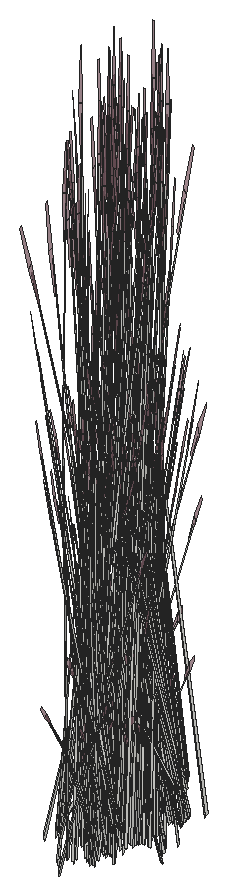
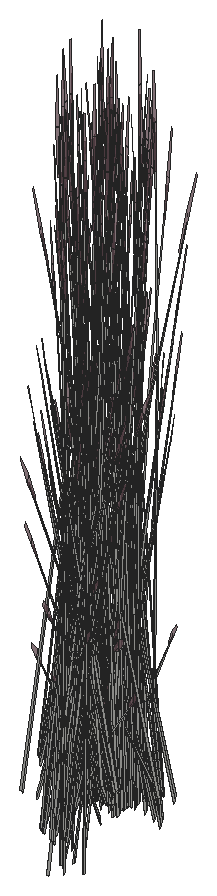
# SketchUp Ruby script. Lengths in inches.
U = 1.inch
M = Sketchup.active_model
def pt(a) = Geom::Point3d.new(a.map { |v| v * U })
def face(e, loops, mat)
  f = e.add_face(loops[0].map { |a| pt(a) })
  loops[1..].each { |l| e.add_face(l.map { |a| pt(a) }).erase! }
  f.material = f.back_material = mat if mat
  f
end
# faces: each face lists its corners as indices into pts; further lists are holes
def faces(e, pts, list, mat = nil) = list.each { |f| face(e, (f[0].is_a?(Array) ? f : [f]).map { |l| l.map { |i| pts[i] } }, mat) }
# xy, xz, yz: faces in a plane at the given z, y or x. An outline is a flat list of corners, or four numbers for a rectangle; further outlines are holes
def ring(l) = l.size == 4 ? [[l[0], l[1]], [l[2], l[1]], [l[2], l[3]], [l[0], l[3]]] : l.each_slice(2).to_a
def flat(e, list, mat, &to3) = list.each { |f| face(e, (f[0].is_a?(Array) ? f : [f]).map { |l| ring(l).map { |u, v| to3.(u, v) } }, mat) }
def xy(e, z, list, mat = nil) = flat(e, list, mat) { |x, y| [x, y, z] }
def xz(e, y, list, mat = nil) = flat(e, list, mat) { |x, z| [x, y, z] }
def yz(e, x, list, mat = nil) = flat(e, list, mat) { |y, z| [x, y, z] }
def lines(e, pts, list) = list.each { |a, b| e.add_line(pt(pts[a]), pt(pts[b])) }
# prism: a flat outline (further loops are holes) pulled along v
def prism(e, loops, v, mat = nil)
  f = face(e, loops, mat); d = Geom::Vector3d.new(v.map { |x| x * U })
  f.pushpull(f.normal.samedirection?(d) ? d.length : -d.length)
end
def box(e, o, s, mat = nil) = prism(e, [[o, [o[0] + s[0], o[1], o[2]], [o[0] + s[0], o[1] + s[1], o[2]], [o[0], o[1] + s[1], o[2]]]], [0, 0, s[2]], mat)
def at(x, y, z, deg = 0) = Geom::Transformation.translation(pt([x, y, z])) * Geom::Transformation.rotation(ORIGIN, Z_AXIS, deg.degrees)
def axes(o, x, y, z) = Geom::Transformation.new([*x, 0, *y, 0, *z, 0, *pt(o).to_a, 1])
def part(name) = M.definitions.add(name)
# library, detail: a bought-in or finely detailed component or shape, given as its bounding box
def library(name, o, s) = part(name).tap { |d| box(d.entities, o, s) }
def detail(e, o, s) = box(e.add_group.entities, o, s)
def put(e, d, t, mat = nil) = e.add_instance(d, t).tap { |i| i.material = mat if mat }
def group(e, t, mat = nil) = e.add_group.tap { |g| g.transformation = t; g.material = mat if mat }.entities
root = M.entities
M.materials.add("LightPink_Translucent").color = [144, 107, 117]
M.materials["LightPink_Translucent"].alpha = 0.75
c1 = part("blade")
p = [[2.15,0.21,22],[0,0.17,0],[0.09,0.45,0],[2.18,0.31,22],[2.29,0.31,22],[0.38,0.45,0],
  [2.48,0.24,33],[2.49,0.24,33],[2.48,0.22,33]]
faces(c1.entities,p,[[0,1,2,3],[4,5,2,3],[6,3,4,7],[8,0,3,6]])
c2 = part("seeds")
p = [[0.3,-0.1,1.38],[-0.01,-0.03,1.59],[-0.01,-0.03,0.03],[0.14,-0.07,-0.07],[0.29,-0.03,3],[0.15,0.01,3.11]]
faces(c2.entities,p,[[0,1,2,3],[1,0,4,5]],"LightPink_Translucent")
c3 = part("blade with seeds")
put(c3.entities,c1,at(0,0,0))
put(c3.entities,c2,axes([2.4,0.25,30.99],[1.5799,-0.05474,1.17369],[-0.12525,1.92788,0.29478],[-0.07173,-0.02425,1.56792]))
put(root,c3,axes([358.98,656.59,622.9],[-0.23773,0.35053,-0.62353],[-0.29532,-0.31785,-0.16365],[-0.09526,0.08744,1.37633]))
put(root,c3,axes([357.93,660.52,622.73],[0.16041,-0.29625,0.0643],[0.22843,0.17248,0.50621],[-0.07385,-0.09498,0.77189]))
put(root,c3,axes([358.37,653.98,625.9],[0.05451,0.37564,0.35414],[-0.31161,0.09919,-0.4572],[-0.0837,-0.10765,0.87481]))
put(root,c3,axes([357.79,654.2,622.64],[-0.2773,-0.3397,0.17642],[0.27945,-0.32949,0.35086],[-0.03063,0.06937,1.60407]))
put(root,c3,axes([357.66,655.44,623.18],[-0.32829,0.39208,0.30756],[-0.32849,-0.38796,-0.36492],[-0.01146,-0.11134,1.64885]))
put(root,c3,axes([356.83,654,622.375],[0,-0.53961,0],[0.44133,0,0],[0,0,1.79456]))
put(root,c3,axes([356.42,654.1,622.6],[0.39767,0.22603,0.24065],[-0.19139,0.46966,0.50002],[0,-0.10827,1.60543]))
put(root,c3,axes([357.05,654.22,622.46],[0,0.53934,-0.05637],[-0.44133,0,0],[0,0.01695,1.79368]))
put(root,c3,axes([359.01,656.53,624.17],[0.305,0.18805,1.51261],[-0.29879,0.40513,0.59816],[-0.13384,-0.24012,1.26806]))
put(root,c3,axes([355.6875,660.78,620.375],[-0.22066,-0.46731,0],[0.36918,-0.26061,-0.51607],[0.08408,-0.05936,1.63711]))
put(root,c3,axes([356.29,653.79,622.89],[-0.38326,0.02879,0.44739],[-0.03466,-0.47788,-0.21531],[0.06861,-0.04843,1.43643]))
put(root,c3,axes([356.27,655.86,625.22],[0.1064,-0.35863,0.35414],[0.31043,0.1046,-0.4572],[0.02846,0.14439,0.87481]))
put(root,c3,axes([357.85,653.12,623.61],[0.18411,0.16231,1.1486],[-0.26813,0.09757,0.84392],[-0.05737,-0.12474,0.25299]))
put(root,c3,axes([359.15,656.4,623.31],[-0.34464,-0.37536,-0.25192],[0.29,-0.42149,0.5513],[-0.0928,0.04391,1.68216]))
put(root,c3,axes([358.52,656.04,623.06],[-0.21202,-0.39143,-0.44739],[0.32115,-0.27564,0.21531],[-0.06861,-0.04843,1.43643]))
put(root,c3,axes([354.45,653.61,623.85],[0.07571,-0.00789,1.74944],[0.20767,-0.36231,-0.27667],[0.13467,0.04783,0.14031]))
put(root,c3,axes([356.11,652.96,622.64],[-0.10196,0.46348,0.17642],[-0.3731,-0.13116,0.35086],[0.06445,-0.00226,1.60407]))
put(root,c3,axes([356.84,655.26,622.46],[0.15345,0.53576,-0.06012],[-0.43845,0.18773,0],[0.00536,0.01871,1.72173]))
put(root,c3,axes([358.28,659.64,622.72],[-0.05398,-0.06539,1.74944],[-0.36026,0.04145,-0.27667],[-0.0575,-0.15639,0.14031]))
put(root,c3,axes([356.61,659.65,620.77],[0.04528,0.27194,1.1486],[-0.25117,-0.15062,0.84392],[0.02703,-0.13924,0.25299]))
put(root,c3,axes([354.53,652.65,623.82],[0.09562,-0.42421,-0.51099],[0.32782,0.1454,-0.3958],[0.13199,-0.0389,0.97773]))
put(root,c3,axes([358.23,653.54,625.9375],[0.39316,-0.11987,0.53763],[0.06823,0.47021,0.4433],[-0.09247,-0.13858,1.11249]))
put(root,c3,axes([355.35,652.93,621.9],[-0.21807,0.07699,1.1486],[0.10265,-0.31819,0.84392],[0.11568,0.02177,0.25299]))
put(root,c3,axes([358.97,656.32,623.06],[-0.38326,0.02879,-0.44739],[-0.03466,-0.47788,0.21531],[-0.06861,0.04843,1.43643]))
put(root,c3,axes([355.93,652.39,622.54],[-0.22066,-0.46731,0],[0.36918,-0.26061,-0.51607],[0.08408,-0.05936,1.63711]))
put(root,c3,axes([358.11,654.56,622.37],[-0.44111,-0.00373,-0.04976],[0,-0.52122,0.49943],[-0.01386,0.11865,1.58352]))
put(root,c3,axes([358.32,653.64,625.58],[0.16041,-0.29625,0.0643],[0.22843,0.17248,0.50621],[-0.07385,-0.09498,0.77189]))
put(root,c3,axes([354.73,652.85,623.66],[0.29332,0.1301,-0.35414],[-0.08555,0.37955,0.4572],[0.11809,-0.0348,0.87481]))
put(root,c3,axes([357.24,652.99,622.64],[-0.37926,0.12378,0.17642],[-0.09365,-0.46065,0.35086],[0.03382,0.06712,1.60407]))
put(root,c3,axes([358.24,657.12,623.32],[0.33032,0.23318,0.49651],[-0.19744,0.41812,0],[-0.07523,-0.05311,1.57504]))
put(root,c3,axes([357.6875,660.09,622.71],[-0.03584,0.03562,1.77383],[-0.35118,-0.12018,-0.16761],[-0.01271,-0.15545,0.31391]))
put(root,c3,axes([357.41,661.12,623.03],[-0.3879,-0.02311,-0.1216],[0.0106,-0.43749,-0.67495],[0.02694,-0.1685,1.02557]))
put(root,c3,axes([354.16,653.67,624.12],[0.35281,0.01123,-0.71045],[-0.0237,0.47284,0.08574],[0.14947,0.0499,1.00501]))
put(root,c3,axes([356.6875,657.14,625.81],[0.2439,-0.26754,-0.06488],[0.22348,0.29302,-0.29416],[0.01573,0.08303,0.97024]))
put(root,c3,axes([358.55,656.26,623.28],[0.09355,-0.55261,-0.23429],[0.44354,0.09633,0.51271],[-0.0775,-0.07631,1.5644]))
put(root,c3,axes([356.62,653.66,622.53],[-0.29264,0.42323,0.45755],[-0.34767,-0.3736,0.17955],[0.07055,-0.04224,1.58856]))
put(root,c3,axes([354.875,652.77,621.12],[-0.22732,0.05597,1.41583],[-0.03618,-0.44548,0.08104],[0.15921,-0.06743,0.80566]))
put(root,c3,axes([357.12,654.33,622.38],[0.24637,0.30123,0],[-0.24637,0.30123,0],[0,0,1.69266]))
put(root,c3,axes([357.12,653.98,622.89],[0.17124,-0.42022,0.44739],[0.35581,0.20224,-0.21531],[0,0.09687,1.43643]))
put(root,c3,axes([356.97,655.4375,622.37],[0.35581,0.20937,0],[-0.17124,0.43505,0],[0,0,1.74954]))
put(root,c3,axes([358.71,656.39,623.46],[-0.06809,0.4162,0.1448],[-0.33266,-0.07225,-0.41347],[-0.06054,-0.04274,1.26744]))
put(root,c3,axes([355.125,652.48,620.63],[-0.01845,-0.0708,1.76342],[0.12793,-0.41416,-0.26939],[0.12905,-0.00596,0.30037]))
put(root,c3,axes([357.875,662.17,620.1],[-0.14494,-0.47823,-0.69835],[0.41752,-0.17223,-0.18329],[-0.01602,-0.16194,1.54149]))
put(root,c3,axes([358.82,660.65,623.03],[-0.34538,0.21713,-0.1216],[-0.16972,-0.38536,-0.67495],[-0.04557,-0.16239,1.02557]))
put(root,c3,axes([358.53,660.66,622.68],[-0.34695,-0.11691,-0.51099],[0.11892,-0.40083,-0.3958],[-0.03181,-0.16138,0.97773]))
put(root,c3,axes([355.25,654.27,623.85],[-0.03191,-0.04083,1.77383],[0.06981,-0.43764,-0.16761],[0.12571,-0.02796,0.31391]))
put(root,c3,axes([357.26,661.19,623.05],[-0.23881,0.24554,0.35414],[-0.22606,-0.28036,-0.4572],[0.0344,-0.14245,0.87481]))
put(root,c3,axes([359.375,657.55,622.86],[-0.33032,0.23318,-0.49651],[-0.19744,-0.41812,0],[-0.07523,0.05311,1.57504]))
put(root,c3,axes([357.42,655.23,622.86],[0,-0.46636,-0.49651],[0.39487,0,0],[0,-0.10622,1.57504]))
put(root,c3,axes([357.59,655.66,623.32],[0,0.46636,0.49651],[-0.39487,0,0],[0,-0.10622,1.57504]))
put(root,c3,axes([359.4,657.43,623.04],[-0.21791,-0.46895,-0.05142],[0.36918,-0.26061,0.51607],[-0.09097,0.04465,1.6363]))
put(root,c3,axes([353.93,652.38,623.01],[-0.14639,0.01056,1.71376],[0.09712,-0.45778,0.13857],[0.20862,0.02831,0.73262]))
put(root,c3,axes([356.46,655.99,624.85],[0.34695,0.11691,-0.51099],[-0.11892,0.40083,-0.3958],[0.03181,0.16138,0.97773]))
put(root,c3,axes([356.17,656.01,625.2],[0.34538,-0.21713,-0.1216],[0.16972,0.38536,-0.67495],[0.04557,0.16239,1.02557]))
put(root,c3,axes([361.12,658.84,626.56],[0.14639,-0.01056,1.71376],[-0.09712,0.45778,0.13857],[-0.20862,-0.02831,0.73262]))
put(root,c3,axes([357.15,660.95,622.68],[-0.25266,-0.31335,-0.51099],[0.2669,-0.27442,-0.3958],[0.03844,-0.15921,0.97773]))
put(root,c3,axes([357,653.875,622.55],[-0.44609,-0.09826,0.49198],[0.09078,-0.55493,0.19306],[0.06519,0.05359,1.70813]))
put(root,c3,axes([358.02,654.63,622.2],[-0.24637,0.29097,-0.30978],[-0.24637,-0.29097,0.30978],[0,0.09372,1.38974]))
put(root,c3,axes([358.3,660.23,620.13],[-0.2439,0.26754,-0.03893],[-0.22348,-0.29302,-0.17649],[-0.01573,-0.08303,0.58215]))
put(root,c3,axes([359.3,657.37,622.875],[-0.32928,-0.11539,-0.30978],[0.08291,-0.40636,0.30978],[-0.06638,0.04686,1.38974]))
put(root,c3,axes([357.88,656.98,625.9],[0.23881,-0.24554,0.35414],[0.22606,0.28036,-0.4572],[-0.0344,0.14245,0.87481]))
put(root,c3,axes([354.46,652.81,624.12],[0.31014,-0.20596,-0.71045],[0.17284,0.42397,0.08574],[0.14985,-0.04816,1.00501]))
put(root,c3,axes([357.3125,654.58,622.26],[0.12941,0.42699,-0.69212],[-0.37279,0.15378,-0.18165],[0.0143,0.14459,1.52773]))
put(root,c3,axes([358.45,655.77,623.51],[-0.39748,-0.22252,-0.29095],[0.19139,-0.46966,-0.50002],[-0.01249,-0.11531,1.59708]))
put(root,c3,axes([359.48,655.63,623.6875],[-0.00964,-0.43909,1.41272],[0.43635,0.11382,0.59816],[-0.1032,0.24027,1.3335]))
put(root,c3,axes([357.13,654.12,622.375],[0.39487,0,0],[0,0.48281,0],[0,0,1.78407]))
put(root,c3,axes([357.5,652.8,625.22],[-0.23881,0.24554,0.35414],[-0.22606,-0.28036,-0.4572],[0.0344,-0.14245,0.87481]))
put(root,c3,axes([356.75,653.59,622.89],[-0.21202,-0.39143,0.44739],[0.32115,-0.27564,-0.21531],[0.06861,0.04843,1.43643]))
put(root,c3,axes([356.36,653.68,622.83],[-0.04113,-0.53214,-0.29095],[0.42835,-0.03218,-0.50002],[0.07543,-0.07088,1.59708]))
put(root,c3,axes([357.27,654.07,622.79],[0.32884,-0.136,0.1448],[0.11516,0.38837,-0.41347],[0,0.08547,1.26744]))
put(root,c3,axes([358.65,660.74,622.98],[-0.16845,-0.3792,-0.71045],[0.34676,-0.21133,0.08574],[-0.03939,-0.18322,1.00501]))
put(root,c3,axes([356.98,660.4,620.59],[-0.10032,0.0944,1.43002],[-0.30046,-0.16522,-0.30754],[0.05569,-0.20547,0.61141]))
put(root,c3,axes([355.51,652.36,623.85],[0.04898,-0.07104,1.74944],[-0.06269,-0.43574,-0.27667],[0.12289,-0.08262,0.14031]))
put(root,c3,axes([359.24,656.1875,623.51],[0.04113,0.53214,-0.29095],[-0.42835,0.03218,-0.50002],[-0.07543,0.07088,1.59708]))
put(root,c3,axes([358.27,655.29,622.94],[-0.14494,-0.47823,-0.69835],[0.41752,-0.17223,-0.18329],[-0.01602,-0.16194,1.54149]))
put(root,c3,axes([359.22,653.77,625.88],[-0.34538,0.21713,-0.1216],[-0.16972,-0.38536,-0.67495],[-0.04557,-0.16239,1.02557]))
put(root,c3,axes([358.92,653.79,625.53],[-0.34695,-0.11691,-0.51099],[0.11892,-0.40083,-0.3958],[-0.03181,-0.16138,0.97773]))
put(root,c3,axes([357.15,654.1,622.83],[0.39748,0.22252,-0.29095],[-0.19139,0.46966,-0.50002],[0.01249,0.11531,1.59708]))
put(root,c3,axes([354.94,653.4375,621.73],[-0.085,-0.1147,1.43002],[0.1106,-0.37943,-0.30754],[0.17198,0.0514,0.61141]))
put(root,c3,axes([356.31,652.5,622.2],[0.32928,0.11539,-0.30978],[-0.08291,0.40636,0.30978],[0.06638,-0.04686,1.38974]))
put(root,c3,axes([358.72,660.8,623.05],[-0.1064,0.35863,0.35414],[-0.31043,-0.1046,-0.4572],[-0.02846,-0.14439,0.87481]))
put(root,c3,axes([357.59,655.24,622.875],[0.24637,-0.29097,-0.30978],[0.24637,0.29097,0.30978],[0,-0.09372,1.38974]))
put(root,c3,axes([358.7,653.36,622.97],[-0.2439,0.26754,-0.03893],[-0.22348,-0.29302,-0.17649],[-0.01573,-0.08303,0.58215]))
put(root,c3,axes([358.6,655.99,623.21],[0.44609,0.09826,0.45755],[-0.09078,0.55493,0.17955],[-0.06519,-0.05359,1.58856]))
put(root,c3,axes([357.23,661.1,622.98],[0.00918,-0.43138,-0.71045],[0.38672,0.02897,0.08574],[0.04081,-0.18275,1.00501]))
put(root,c3,axes([358.02,654.21,622.65],[0,-0.46636,0.49651],[0.39487,0,0],[0,0.10622,1.57504]))
put(root,c3,axes([358.1875,654.64,622.1875],[0,0.46636,-0.49651],[-0.39487,0,0],[0,0.10622,1.57504]))
put(root,c3,axes([357.13,656.06,624.9],[-0.35104,0.10702,0.48003],[-0.06092,-0.41983,0.3958],[0.08256,0.12373,0.9933]))
put(root,c3,axes([356.23,652.32,622.1875],[0.33032,-0.23318,-0.49651],[0.19744,0.41812,0],[0.07523,-0.05311,1.57504]))
put(root,c3,axes([357.06,656.14,624.9],[-0.16041,0.29625,0.0643],[-0.22843,-0.17248,0.50621],[0.07385,0.09498,0.77189]))
put(root,c3,axes([356.66,655.16,624.04],[-0.08068,-0.14973,1.71376],[0.3728,-0.12606,0.13857],[0.08426,0.23506,0.73262]))
put(root,c3,axes([356.89,653.48,622.79],[0.06809,-0.4162,0.1448],[0.33266,0.07225,-0.41347],[0.06054,0.04274,1.26744]))
put(root,c3,axes([358.49,655.89,623.5625],[-0.17124,0.42022,0.44739],[-0.35581,-0.20224,-0.21531],[0,-0.09687,1.43643]))
put(root,c3,axes([357.37,652.75,622.65],[-0.33032,-0.23318,0.49651],[0.19744,-0.41812,0],[0.07523,0.05311,1.57504]))
put(root,c3,axes([358.36,659.9,619.49],[-0.0592,0.0168,1.76342],[-0.32738,-0.18913,-0.26939],[0.00549,-0.15776,0.30037]))
put(root,c3,axes([358.36,656.88,623.32],[0.37926,-0.12378,0.17642],[0.09365,0.46065,0.35086],[-0.03382,-0.06712,1.60407]))
put(root,c3,axes([361.55,658.41,627.66],[-0.35281,-0.01123,-0.71045],[0.0237,-0.47284,0.08574],[-0.14947,-0.0499,1.00501]))
put(root,c3,axes([358.85,656.95,623.04],[-0.35581,-0.20937,0],[0.17124,-0.43505,0],[0,0,1.62707]))
put(root,c3,axes([357.08,655.19,622.35],[0.37054,-0.15823,-0.19198],[0.1302,0.45581,0.00008],[0.0409,-0.01749,1.73897]))
put(root,c3,axes([359.12,653.93,625.9],[-0.1064,0.35863,0.35414],[-0.31043,-0.1046,-0.4572],[-0.02846,-0.14439,0.87481]))
put(root,c3,axes([361.27,658.53,625.27],[0.06891,0.12984,1.43002],[-0.15879,0.35293,-0.30754],[-0.16304,-0.08436,0.61141]))
put(root,c3,axes([358.6875,660.42,622.53],[0.1064,-0.35863,-0.35414],[0.31043,0.1046,0.4572],[-0.02846,-0.14439,0.87481]))
put(root,c3,axes([359.67,657.48,623.22],[0.22066,0.46731,0],[-0.36918,0.26061,-0.51607],[-0.08408,0.05936,1.63711]))
put(root,c3,axes([357.39,660.84,622.53],[0.23881,-0.24554,-0.35414],[0.22606,0.28036,0.4572],[0.0344,-0.14245,0.87481]))
put(root,c3,axes([357.48,660.96,622.73],[0.29004,0.02173,0.0643],[-0.00795,0.32812,0.50621],[0.03035,-0.12569,0.77189]))
put(root,c3,axes([361.39,658.1,626.56],[0.1311,0.08035,1.71376],[-0.27131,0.33708,0.13857],[-0.16909,-0.15206,0.73262]))
put(root,c3,axes([357.77,660.42,622.72],[-0.00341,-0.09282,1.74944],[-0.28775,-0.26825,-0.27667],[0.04449,-0.16261,0.14031]))
put(root,c3,axes([357.02,655.8,625.22],[-0.05451,-0.37564,0.35414],[0.31161,-0.09919,-0.4572],[0.0837,0.10765,0.87481]))
put(root,c3,axes([357.39,660.93,622.73],[0.25132,0.3182,0.48003],[-0.2669,0.27442,0.3958],[0.04636,-0.14929,0.9933]))
put(root,c3,axes([359.49,656.91,623.32],[0.10196,-0.46348,0.17642],[0.3731,0.13116,0.35086],[-0.06445,0.00226,1.60407]))
put(root,c3,axes([359.32,656.29,623.46],[0.26075,0.2802,0.1448],[-0.2175,0.31612,-0.41347],[-0.06054,0.04274,1.26744]))
put(root,c3,axes([357.08,653.83,622.38],[0.21202,0.39143,-0.44739],[-0.32115,0.27564,0.21531],[0.06861,0.04843,1.43643]))
put(root,c3,axes([359.23,655.95,623.14],[-0.32829,-0.4014,-0.06131],[0.32849,-0.40164,0],[-0.01146,-0.01402,1.75571]))
put(root,c3,axes([359.3125,656.09,623.5625],[0.38326,-0.02879,0.44739],[0.03466,0.47788,-0.21531],[-0.06861,0.04843,1.43643]))
put(root,c3,axes([357.22,653.64,624.64],[-0.30498,-0.24231,1.38283],[0.32203,-0.37727,0.59665],[0.0984,0.22736,1.33663]))
put(root,c3,axes([361.4375,658.51,627.36],[-0.25628,0.30892,-0.51099],[-0.22444,-0.32634,-0.3958],[-0.13021,-0.047,0.97773]))
put(root,c3,axes([356.71,656.33,624.88],[0.00104,-0.05646,1.77383],[0.30246,-0.2491,-0.16761],[0.10506,0.08891,0.31391]))
put(root,c3,axes([361.02,659.4,624.17],[0.00895,0.0735,1.76342],[-0.18044,0.38382,-0.26939],[-0.12817,-0.01935,0.30037]))
put(root,c3,axes([357.72,652.58,624.9],[0.29004,0.02173,0.0643],[-0.00795,0.32812,0.50621],[0.03035,-0.12569,0.77189]))
put(root,c3,axes([359.4,657.18,623.18],[0.44186,0.15158,0.30756],[-0.11054,0.54181,-0.36492],[-0.07313,0.06781,1.64885]))
put(root,c3,axes([357.68,655.61,622.93],[-0.19872,-0.13409,1.1486],[0.2566,-0.13625,0.84392],[0.06921,0.11541,0.25299]))
put(root,c3,axes([356.98,655.47,622.76],[0.00623,-0.15459,1.43002],[0.29764,-0.17268,-0.30754],[0.09188,0.18503,0.61141]))
put(root,c3,axes([359.6,657.15,623.32],[0.33032,-0.23318,0.49651],[0.19744,0.41812,0],[-0.07523,0.05311,1.57504]))
put(root,c3,axes([356.62,653.28,622.23],[0.23773,-0.35053,-0.62353],[0.29532,0.31785,-0.16365],[0.09526,-0.08744,1.37633]))
put(root,c3,axes([358.82,660.47,622.73],[0.26007,-0.1585,0.0643],[0.12729,0.28902,0.50621],[-0.02512,-0.1274,0.77189]))
put(root,c3,axes([357.625,652.55,624.9],[0.25132,0.3182,0.48003],[-0.2669,0.27442,0.3958],[0.04636,-0.14929,0.9933]))
put(root,c3,axes([361.08,657.64,627.39],[0.02617,0.04654,1.77383],[-0.12614,0.41836,-0.16761],[-0.12775,0.00303,0.31391]))
put(root,c3,axes([359.08,653.55,625.37],[0.1064,-0.35863,-0.35414],[0.31043,0.1046,0.4572],[-0.02846,-0.14439,0.87481]))
put(root,c3,axes([358.5625,655.48,623.21],[0.15345,0.52148,0.45755],[-0.43845,0.18134,0.17955],[0.00536,-0.09582,1.58856]))
put(root,c3,axes([358.49,655.42,623.06],[0.17124,-0.42022,-0.44739],[0.35581,0.20224,0.21531],[0,-0.09687,1.43643]))
put(root,c3,axes([358.72,660.5,622.73],[0.34777,0.12192,0.48003],[-0.11892,0.40083,0.3958],[-0.0209,-0.15763,0.9933]))
put(root,c3,axes([358.93,656.77,623.05],[-0.11516,-0.40207,0],[0.32884,-0.1408,0],[0,0,1.54371]))
put(root,c3,axes([361.37,657.36,627.4],[-0.07594,-0.00329,1.74944],[-0.24177,0.32918,-0.27667],[-0.129,-0.06726,0.14031]))
put(root,c3,axes([356.79,660.88,621.875],[-0.06572,0.16029,1.71376],[-0.27569,-0.33172,0.13857],[0.12437,-0.20675,0.73262]))
put(root,c3,axes([357.67,652.97,622.2],[0.08291,0.40636,-0.30978],[-0.32928,0.11539,0.30978],[0.06638,0.04686,1.38974]))
put(root,c3,axes([358.28,654.29,622.55],[0.44133,0,0],[0,0.52122,-0.51607],[0,0.11871,1.63711]))
put(root,c3,axes([361.06,659.18,627.41],[0.09971,-0.42522,0.48003],[0.32782,0.1454,0.3958],[-0.12892,0.02555,0.9933]))
put(root,c3,axes([361.57,658.18,627.71],[-0.0189,0.47427,-0.1216],[-0.35781,-0.01296,-0.67495],[-0.13781,-0.03295,1.02557]))
put(root,c3,axes([361.34,658.22,627.21],[-0.20082,-0.29199,-0.35414],[0.2293,-0.2764,0.4572],[-0.1165,-0.04206,0.87481]))
put(root,c3,axes([361.03,659.07,627.41],[-0.12963,-0.31798,0.0643],[0.23638,-0.15564,0.50621],[-0.1042,0.03071,0.77189]))
put(root,c3,axes([356.86,653.61,622.83],[0.35635,-0.30962,-0.29095],[0.23697,0.43749,-0.50002],[0.08792,0.04443,1.59708]))
put(root,c3,axes([357.72,656.22,622.84],[-0.22633,-0.01463,1.0506],[0.14947,-0.31064,0.58006],[0.08941,0.11036,0.8241]))
put(root,c3,axes([357.92,653.5625,625.22],[-0.30722,0.06665,0.35414],[-0.08112,-0.381,-0.4572],[0.08804,-0.10234,0.87481]))
put(root,c3,axes([357.84,661.98,623.03],[-0.32648,-0.25715,-0.1216],[0.18809,-0.3724,-0.67495],[0.09224,-0.12945,1.02557]))
put(root,c3,axes([359.4,655.98,623.06],[-0.17124,0.42022,-0.44739],[-0.35581,-0.20224,0.21531],[0,0.09687,1.43643]))
put(root,c3,axes([357.82,660.79,620.375],[-0.22066,-0.46731,0],[0.36918,-0.26061,-0.51607],[0.08408,-0.05936,1.63711]))
put(root,c3,axes([360.86,658.92,625.45],[0.22533,-0.03337,1.1486],[-0.14293,0.29403,0.84392],[-0.11135,-0.04411,0.25299]))
put(root,c3,axes([359.21,653.6,625.58],[0.26007,-0.1585,0.0643],[0.12729,0.28902,0.50621],[-0.02512,-0.1274,0.77189]))
put(root,c3,axes([360.07,655.72,623.32],[-0.2773,-0.3397,0.17642],[0.27945,-0.32949,0.35086],[-0.03063,0.06937,1.60407]))
put(root,c3,axes([359.11,655.53,623.05],[0,-0.53961,0],[0.44133,0,0],[0,0,1.79456]))
put(root,c3,axes([359.12,653.63,625.58],[0.34777,0.12192,0.48003],[-0.11892,0.40083,0.3958],[-0.0209,-0.15763,0.9933]))
put(root,c3,axes([357.68,660.6875,619.49],[-0.05283,-0.03674,1.76342],[-0.13569,-0.41045,-0.26939],[0.09154,-0.11138,0.30037]))
put(root,c3,axes([358.7,655.625,623.28],[0.39767,0.22603,0.24065],[-0.19139,0.46966,0.50002],[0,-0.10827,1.60543]))
put(root,c3,axes([358.74,659.66,620.77],[0.04528,0.27194,1.1486],[-0.25117,-0.15062,0.84392],[0.02703,-0.13924,0.25299]))
put(root,c3,axes([359.34,655.74,623.14],[0,0.53934,-0.05637],[-0.44133,0,0],[0,0.01695,1.79368]))
put(root,c3,axes([358.58,655.3125,623.5625],[-0.38326,0.02879,0.44739],[-0.03466,-0.47788,-0.21531],[0.06861,-0.04843,1.43643]))
put(root,c3,axes([356.99,655.99,625.2],[0.21031,-0.39918,-0.1216],[0.30457,0.22997,-0.67495],[0.10587,0.11278,1.02557]))
put(root,c3,axes([355.96,653.34,621.76],[-0.3474,0.18671,1.28929],[-0.11057,-0.53572,0.50096],[0.21332,0.00891,1.46642]))
put(root,c3,axes([361.3125,658.11,627.77],[0.29147,-0.34417,0.53763],[0.25138,0.3655,0.4433],[-0.13675,-0.06349,1.11249]))
put(root,c3,axes([358.08,653.6,625.2],[-0.32648,-0.25715,-0.1216],[0.18809,-0.3724,-0.67495],[0.09224,-0.12945,1.02557]))
put(root,c3,axes([358.4,654.49,623.32],[-0.10196,0.46348,0.17642],[-0.3731,-0.13116,0.35086],[0.06445,-0.00226,1.60407]))
put(root,c3,axes([359.125,656.79,623.14],[0.15345,0.53576,-0.06012],[-0.43845,0.18773,0],[0.00536,0.01871,1.72173]))
put(root,c3,axes([357.67,661.67,622.68],[-0.09067,-0.42583,-0.51099],[0.34336,-0.07449,-0.3958],[0.0984,-0.11438,0.97773]))
put(root,c3,axes([357.24,655.8,624.85],[0.34827,-0.11086,-0.51099],[0.06092,0.41983,-0.3958],[0.09354,0.12031,0.97773]))
put(root,c3,axes([359.82,660.11,622.71],[-0.03584,0.03562,1.77383],[-0.35118,-0.12018,-0.16761],[-0.01271,-0.15545,0.31391]))
put(root,c3,axes([359.54,661.13,623.03],[-0.3879,-0.02311,-0.1216],[0.0106,-0.43749,-0.67495],[0.02694,-0.1685,1.02557]))
put(root,c3,axes([357.56,652.51,622.55],[0.22066,-0.46731,0],[0.36918,0.26061,-0.51607],[0.08408,0.05936,1.63711]))
put(root,c3,axes([358.21,653.92,623.22],[-0.22066,-0.46731,0],[0.36918,-0.26061,-0.51607],[0.08408,-0.05936,1.63711]))
put(root,c3,axes([357.64,655.29,625.22],[-0.20082,-0.29199,0.35414],[0.2293,-0.2764,-0.4572],[0.1165,0.04206,0.87481]))
put(root,c3,axes([360.39,656.08,623.04],[-0.44111,-0.00373,-0.04976],[0,-0.52122,0.49943],[-0.01386,0.11865,1.58352]))
put(root,c3,axes([357.76,652.79,622.1875],[0.33032,0.23318,-0.49651],[-0.19744,0.41812,0],[0.07523,0.05311,1.57504]))
put(root,c3,axes([359.53,654.52,623.32],[-0.37926,0.12378,0.17642],[-0.09365,-0.46065,0.35086],[0.03382,0.06712,1.60407]))
put(root,c3,axes([357.82,655.56,624.9],[-0.01777,0.35463,0.0643],[-0.26836,-0.00972,0.50621],[0.1028,0.03711,0.77189]))
put(root,c3,axes([359.39,661.2,623.05],[-0.23881,0.24554,0.35414],[-0.22606,-0.28036,-0.4572],[0.0344,-0.14245,0.87481]))
put(root,c3,axes([357.74,656.11,621.66],[0.02571,-0.06733,1.76342],[0.32373,-0.19829,-0.26939],[0.09815,0.10263,0.30037]))
put(root,c3,axes([357.84,655.44,624.9],[-0.26024,0.30729,0.48003],[-0.22444,-0.32634,0.3958],[0.1221,0.05668,0.9933]))
put(root,c3,axes([357.91,653.29,624.85],[-0.09067,-0.42583,-0.51099],[0.34336,-0.07449,-0.3958],[0.0984,-0.11438,0.97773]))
put(root,c3,axes([359.14,652.79,623.61],[0.04528,0.27194,1.1486],[-0.25117,-0.15062,0.84392],[0.02703,-0.13924,0.25299]))
put(root,c3,axes([359.28,660.97,622.68],[-0.25266,-0.31335,-0.51099],[0.2669,-0.27442,-0.3958],[0.03844,-0.15921,0.97773]))
put(root,c3,axes([361.45,658.1,627.41],[0.01777,-0.35463,0.0643],[0.26836,0.00972,0.50621],[-0.1028,-0.03711,0.77189]))
put(root,c3,axes([358.91,655.1875,623.21],[-0.29264,0.42323,0.45755],[-0.34767,-0.3736,0.17955],[0.07055,-0.04224,1.58856]))
put(root,c3,axes([358.52,655.49,624.1],[-0.06755,-0.39203,-0.03492],[0.31928,-0.09013,-0.15832],[0.06667,0.02485,0.52218]))
put(root,c3,axes([357.97,654.47,625.22],[-0.29332,-0.1301,0.35414],[0.08555,-0.37955,-0.4572],[0.11809,-0.0348,0.87481]))
put(root,c3,axes([362.2,660.0625,624.74],[-0.36714,-0.07646,-0.62353],[0.07747,-0.47163,-0.16365],[-0.10956,-0.05715,1.37633]))
put(root,c3,axes([359.41,655.86,623.06],[0.24637,0.30123,0],[-0.24637,0.30123,0],[0,0,1.69266]))
put(root,c3,axes([362.27,657.49,628.11],[-0.23555,0.44708,-0.13619],[-0.34112,-0.25757,-0.75594],[-0.11858,-0.12631,1.14864]))
put(root,c3,axes([359.4,655.5,623.5625],[0.17124,-0.42022,0.44739],[0.35581,0.20224,-0.21531],[0,0.09687,1.43643]))
put(root,c3,axes([359.25,656.96,623.05],[0.35581,0.20937,0],[-0.17124,0.43505,0],[0,0,1.74954]))
put(root,c3,axes([361.63,658.37,627.73],[0.20082,0.29199,0.35414],[-0.2293,0.2764,-0.4572],[-0.1165,-0.04206,0.87481]))
put(root,c3,axes([357.28,653.68,622.23],[0.36714,0.07646,-0.62353],[-0.07747,0.47163,-0.16365],[0.10956,0.05715,1.37633]))
put(root,c3,axes([358.84,653.96,622.43],[-0.21881,-0.29821,-0.06488],[0.23965,-0.27324,-0.29416],[0.0679,-0.01924,0.97024]))
put(root,c3,axes([362.17,657.85,627.66],[-0.30095,-0.22541,-0.71045],[0.21388,-0.395,0.08574],[-0.10904,-0.13459,1.00501]))
put(root,c3,axes([362.03,657.86,627.36],[-0.34827,0.11086,-0.51099],[-0.06092,-0.41983,-0.3958],[-0.09354,-0.12031,0.97773]))
put(root,c3,axes([359.29,655.4,623.23],[-0.44609,-0.09826,0.49198],[0.09078,-0.55493,0.19306],[0.06519,0.05359,1.70813]))
put(root,c3,axes([360.21,653.23,625.55],[-0.03584,0.03562,1.77383],[-0.35118,-0.12018,-0.16761],[-0.01271,-0.15545,0.31391]))
